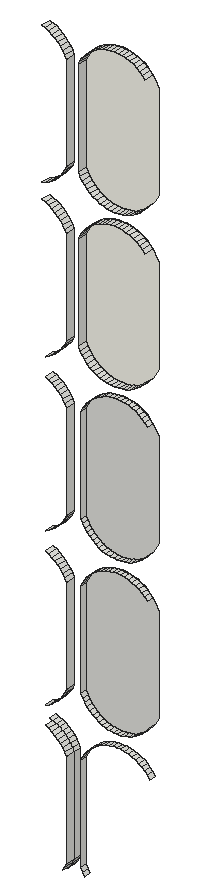
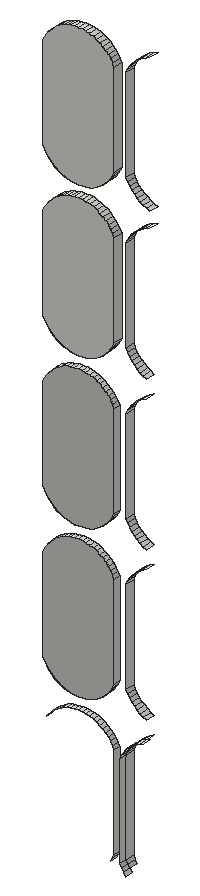
# SketchUp Ruby script. Lengths in inches.
U = 1.inch
M = Sketchup.active_model
def pt(a) = Geom::Point3d.new(a.map { |v| v * U })
def face(e, loops, mat)
  f = e.add_face(loops[0].map { |a| pt(a) })
  loops[1..].each { |l| e.add_face(l.map { |a| pt(a) }).erase! }
  f.material = f.back_material = mat if mat
  f
end
# faces: each face lists its corners as indices into pts; further lists are holes
def faces(e, pts, list, mat = nil) = list.each { |f| face(e, (f[0].is_a?(Array) ? f : [f]).map { |l| l.map { |i| pts[i] } }, mat) }
# xy, xz, yz: faces in a plane at the given z, y or x. An outline is a flat list of corners, or four numbers for a rectangle; further outlines are holes
def ring(l) = l.size == 4 ? [[l[0], l[1]], [l[2], l[1]], [l[2], l[3]], [l[0], l[3]]] : l.each_slice(2).to_a
def flat(e, list, mat, &to3) = list.each { |f| face(e, (f[0].is_a?(Array) ? f : [f]).map { |l| ring(l).map { |u, v| to3.(u, v) } }, mat) }
def xy(e, z, list, mat = nil) = flat(e, list, mat) { |x, y| [x, y, z] }
def xz(e, y, list, mat = nil) = flat(e, list, mat) { |x, z| [x, y, z] }
def yz(e, x, list, mat = nil) = flat(e, list, mat) { |y, z| [x, y, z] }
def lines(e, pts, list) = list.each { |a, b| e.add_line(pt(pts[a]), pt(pts[b])) }
# prism: a flat outline (further loops are holes) pulled along v
def prism(e, loops, v, mat = nil)
  f = face(e, loops, mat); d = Geom::Vector3d.new(v.map { |x| x * U })
  f.pushpull(f.normal.samedirection?(d) ? d.length : -d.length)
end
def box(e, o, s, mat = nil) = prism(e, [[o, [o[0] + s[0], o[1], o[2]], [o[0] + s[0], o[1] + s[1], o[2]], [o[0], o[1] + s[1], o[2]]]], [0, 0, s[2]], mat)
def at(x, y, z, deg = 0) = Geom::Transformation.translation(pt([x, y, z])) * Geom::Transformation.rotation(ORIGIN, Z_AXIS, deg.degrees)
def axes(o, x, y, z) = Geom::Transformation.new([*x, 0, *y, 0, *z, 0, *pt(o).to_a, 1])
def part(name) = M.definitions.add(name)
# library, detail: a bought-in or finely detailed component or shape, given as its bounding box
def library(name, o, s) = part(name).tap { |d| box(d.entities, o, s) }
def detail(e, o, s) = box(e.add_group.entities, o, s)
def put(e, d, t, mat = nil) = e.add_instance(d, t).tap { |i| i.material = mat if mat }
def group(e, t, mat = nil) = e.add_group.tap { |g| g.transformation = t; g.material = mat if mat }.entities
root = M.entities
M.materials.add("Tafisa-Gardenia-or-Gardenia-PM775-4K").color = [246, 245, 235]
xz(root,138.79,[[89.53,63,89.85,63.02,90.17,63.0625,90.48,63.14,90.78,63.25,91.07,63.38,91.35,63.55,91.61,63.73,91.84,63.95,92.0625,64.18,92.25,64.4375,92.42,64.71,92.5625,65,92.5625,73,92.42,73.29,92.25,73.5625,92.0625,73.82,91.84,74.05,91.61,74.27,91.35,74.45,91.07,74.62,90.78,74.75,90.48,74.86,90.17,74.9375,89.85,74.98,89.53,75,89.21,74.98,88.89,74.9375,88.58,74.86,88.28,74.75,87.99,74.62,87.72,74.45,87.46,74.27,87.22,74.05,87,73.82,86.81,73.5625,86.64,73.29,86.5,73,86.5,65,86.64,64.71,86.81,64.4375,87,64.18,87.22,63.95,87.46,63.73,87.72,63.55,87.99,63.38,88.28,63.25,88.58,63.14,88.89,63.0625,89.21,63.02],[89.53,76,89.85,76.02,90.17,76.0625,90.48,76.14,90.78,76.25,91.07,76.38,91.35,76.55,91.61,76.73,91.84,76.95,92.0625,77.18,92.25,77.4375,92.42,77.71,92.5625,78,92.5625,86,92.42,86.29,92.25,86.5625,92.0625,86.82,91.84,87.05,91.61,87.27,91.35,87.45,91.07,87.62,90.78,87.75,90.48,87.86,90.17,87.9375,89.85,87.98,89.53,88,89.21,87.98,88.89,87.9375,88.58,87.86,88.28,87.75,87.99,87.62,87.72,87.45,87.46,87.27,87.22,87.05,87,86.82,86.81,86.5625,86.64,86.29,86.5,86,86.5,78,86.64,77.71,86.81,77.4375,87,77.18,87.22,76.95,87.46,76.73,87.72,76.55,87.99,76.38,88.28,76.25,88.58,76.14,88.89,76.0625,89.21,76.02]])
xz(root,138.79,[[89.53,89,89.85,89.02,90.17,89.0625,90.48,89.14,90.78,89.25,91.07,89.38,91.35,89.55,91.61,89.73,91.84,89.95,92.0625,90.18,92.25,90.4375,92.42,90.71,92.5625,91,92.5625,99,92.42,99.29,92.25,99.5625,92.0625,99.82,91.84,100.05,91.61,100.27,91.35,100.45,91.07,100.62,90.78,100.75,90.48,100.86,90.17,100.9375,89.85,100.98,89.53,101,89.21,100.98,88.89,100.9375,88.58,100.86,88.28,100.75,87.99,100.62,87.72,100.45,87.46,100.27,87.22,100.05,87,99.82,86.81,99.5625,86.64,99.29,86.5,99,86.5,91,86.64,90.71,86.81,90.4375,87,90.18,87.22,89.95,87.46,89.73,87.72,89.55,87.99,89.38,88.28,89.25,88.58,89.14,88.89,89.0625,89.21,89.02],[89.53,102,89.85,102.02,90.17,102.0625,90.48,102.14,90.78,102.25,91.07,102.38,91.35,102.55,91.61,102.73,91.84,102.95,92.0625,103.18,92.25,103.4375,92.42,103.71,92.5625,104,92.5625,112,92.42,112.29,92.25,112.5625,92.0625,112.82,91.84,113.05,91.61,113.27,91.35,113.45,91.07,113.62,90.78,113.75,90.48,113.86,90.17,113.9375,89.85,113.98,89.53,114,89.21,113.98,88.89,113.9375,88.58,113.86,88.28,113.75,87.99,113.62,87.72,113.45,87.46,113.27,87.22,113.05,87,112.82,86.81,112.5625,86.64,112.29,86.5,112,86.5,104,86.64,103.71,86.81,103.4375,87,103.18,87.22,102.95,87.46,102.73,87.72,102.55,87.99,102.38,88.28,102.25,88.58,102.14,88.89,102.0625,89.21,102.02]],"Tafisa-Gardenia-or-Gardenia-PM775-4K")
yz(root,85.5,[[138,52,138.79,60],[138.79,52,139.4375,60],[138,65,138.79,73],[138,78,138.79,86],[138,91,138.79,99],
  [138,104,138.79,112]])
yz(root,86.5,[[138.25,52,138.79,60],[138.25,65,138.79,73],[138.25,78,138.79,86],[138,91,138.79,99],[138,104,138.79,112]])
p = [[85.01,139.4375,51.18],[85.01,138.79,51.18],[85.2,138.79,51.44],[85.2,139.4375,51.44],[85.36,138.79,51.71],[85.2,138,51.44],
  [85.36,138,51.71],[86.81,138.79,51.4375],[86.64,138.79,51.71],[86.64,138.25,51.71],[86.81,138.25,51.4375],[85.36,139.4375,51.71],
  [85.5,138.79,52],[85.5,138,52],[86.5,138.79,52],[86.5,138.25,52],[85.5,139.4375,52],[85.36,138.79,60.29],
  [85.5,138.79,60],[85.5,138,60],[85.36,138,60.29],[86.5,138.79,60],[86.64,138.79,60.29],[86.64,138.25,60.29],
  [86.5,138.25,60],[85.5,139.4375,60],[85.36,139.4375,60.29],[85.2,138.79,60.56],[85.2,138,60.56],[86.81,138.79,60.5625],
  [86.81,138.25,60.5625],[85.2,139.4375,60.56],[85.01,138.79,60.82],[85.01,138,60.82],[87,138.79,60.82],[87,138.25,60.82],
  [92.0625,138.79,60.82],[92.25,138.79,60.5625],[92.25,138.25,60.5625],[92.0625,138.25,60.82],[85.01,139.4375,60.82],[84.79,138.79,61.05],
  [84.79,138,61.05],[87.22,138.79,61.05],[87.22,138.25,61.05],[91.84,138.79,61.05],[91.84,138.25,61.05],[84.79,139.4375,61.05],
  [84.56,138.79,61.26],[84.56,138,61.26],[87.46,138.79,61.27],[87.46,138.25,61.27],[91.61,138.79,61.27],[91.61,138.25,61.27],
  [84.56,139.4375,61.26],[84.3,138.79,61.45],[84.3,138,61.45],[87.72,138.79,61.45],[87.72,138.25,61.45],[91.35,138.79,61.45],
  [91.35,138.25,61.45],[84.3,139.4375,61.45],[84.03,138.79,61.62],[84.03,138,61.62],[87.99,138.79,61.62],[87.99,138.25,61.62],
  [91.07,138.79,61.62],[91.07,138.25,61.62],[84.03,139.4375,61.62],[83.74,138.79,61.75],[83.74,138,61.75],[88.28,138.79,61.75],
  [88.28,138.25,61.75],[90.78,138.79,61.75],[90.78,138.25,61.75],[83.74,139.4375,61.75],[88.58,138.79,61.86],[88.58,138.25,61.86],
  [90.48,138.79,61.86],[90.48,138.25,61.86],[83.44,138.79,61.86],[83.44,139.4375,61.86],[88.89,138.79,61.9375],[88.89,138.25,61.9375],
  [89.21,138.79,61.98],[89.21,138.25,61.98],[89.02,138.25,61.96],[89.85,138.79,61.98],[90.17,138.79,61.9375],[90.17,138.25,61.9375],
  [89.85,138.25,61.98],[89.53,138.79,62],[89.53,138.25,62],[89.21,138.79,63.02],[88.89,138.79,63.0625],[88.89,138.25,63.0625],
  [89.02,138.25,63.04],[89.21,138.25,63.02],[89.53,138.79,63],[89.53,138.25,63],[89.85,138.79,63.02],[89.85,138.25,63.02],
  [90.17,138.79,63.0625],[90.17,138.25,63.0625],[88.58,138.79,63.14],[88.28,138.79,63.25],[88.28,138.25,63.25],[88.58,138.25,63.14],
  [88.78,138.25,63.09],[90.48,138.79,63.14],[90.48,138.25,63.14],[90.78,138.79,63.25],[90.78,138.25,63.25],[84.03,138.79,63.38],
  [83.74,138.79,63.25],[83.74,138,63.25],[84.03,138,63.38],[87.99,138.79,63.38],[87.99,138.25,63.38],[91.07,138.79,63.38],
  [91.07,138.25,63.38],[84.3,138.79,63.55],[84.3,138,63.55],[87.72,138.79,63.55],[87.72,138.25,63.55],[91.35,138.79,63.55],
  [91.35,138.25,63.55],[84.56,138.79,63.74],[84.56,138,63.74],[87.46,138.79,63.73],[87.46,138.25,63.73],[91.61,138.79,63.73],
  [91.61,138.25,63.73],[84.79,138.79,63.95],[84.79,138,63.95],[87.22,138.79,63.95],[87.22,138.25,63.95],[91.84,138.79,63.95],
  [91.84,138.25,63.95],[85.01,138.79,64.18],[85.01,138,64.18],[87,138.79,64.18],[87,138.25,64.18],[92.0625,138.79,64.18],
  [92.0625,138.25,64.18],[85.2,138.79,64.44],[85.2,138,64.44],[86.81,138.79,64.4375],[86.81,138.25,64.4375],[92.25,138.79,64.4375],
  [92.25,138.25,64.4375],[85.36,138.79,64.71],[85.36,138,64.71],[86.64,138.79,64.71],[86.64,138.25,64.71],[85.5,138.79,65],
  [85.5,138,65],[86.5,138.79,65],[86.5,138.25,65],[85.36,138.79,73.29],[85.5,138.79,73],[85.5,138,73],
  [85.36,138,73.29],[86.5,138.79,73],[86.64,138.79,73.29],[86.64,138.25,73.29],[86.5,138.25,73],[85.2,138.79,73.56],
  [85.2,138,73.56],[86.81,138.79,73.5625],[86.81,138.25,73.5625],[85.01,138.79,73.82],[85.01,138,73.82],[87,138.79,73.82],
  [87,138.25,73.82],[84.79,138.79,74.05],[84.79,138,74.05],[87.22,138.79,74.05],[87.22,138.25,74.05],[91.84,138.79,74.05],
  [92.0625,138.79,73.82],[92.0625,138.25,73.82],[91.84,138.25,74.05],[84.56,138.79,74.26],[84.56,138,74.26],[87.46,138.79,74.27],
  [87.46,138.25,74.27],[91.61,138.79,74.27],[91.61,138.25,74.27],[84.3,138.79,74.45],[84.3,138,74.45],[87.72,138.79,74.45],
  [87.72,138.25,74.45],[91.35,138.79,74.45],[91.35,138.25,74.45],[84.03,138.79,74.62],[84.03,138,74.62],[87.99,138.79,74.62],
  [87.99,138.25,74.62],[91.07,138.79,74.62],[91.07,138.25,74.62],[83.74,138.79,74.75],[83.74,138,74.75],[88.28,138.79,74.75],
  [88.28,138.25,74.75],[90.78,138.79,74.75],[90.78,138.25,74.75],[88.58,138.79,74.86],[88.58,138.25,74.86],[90.48,138.79,74.86],
  [90.48,138.25,74.86],[88.89,138.79,74.9375],[88.89,138.25,74.9375],[89.21,138.79,74.98],[89.21,138.25,74.98],[89.02,138.25,74.96],
  [89.85,138.79,74.98],[90.17,138.79,74.9375],[90.17,138.25,74.9375],[89.85,138.25,74.98],[89.53,138.79,75],[89.53,138.25,75],
  [89.21,138.79,76.02],[88.89,138.79,76.0625],[88.89,138.25,76.0625],[89.02,138.25,76.04],[89.21,138.25,76.02],[89.53,138.79,76],
  [89.53,138.25,76],[89.85,138.79,76.02],[89.85,138.25,76.02],[90.17,138.79,76.0625],[90.17,138.25,76.0625],[88.58,138.79,76.14],
  [88.28,138.79,76.25],[88.28,138.25,76.25],[88.58,138.25,76.14],[90.48,138.79,76.14],[90.48,138.25,76.14],[90.78,138.79,76.25],
  [90.78,138.25,76.25],[84.03,138.79,76.38],[83.74,138.79,76.25],[83.74,138,76.25],[84.03,138,76.38],[87.99,138.79,76.38],
  [87.99,138.25,76.38],[91.07,138.79,76.38],[91.07,138.25,76.38],[84.3,138.79,76.55],[84.3,138,76.55],[87.72,138.79,76.55],
  [87.72,138.25,76.55],[91.35,138.79,76.55],[91.35,138.25,76.55],[84.56,138.79,76.74],[84.56,138,76.74],[87.46,138.79,76.73],
  [87.46,138.25,76.73],[91.61,138.79,76.73],[91.61,138.25,76.73],[84.79,138.79,76.95],[84.79,138,76.95],[87.22,138.79,76.95],
  [87.22,138.25,76.95],[91.84,138.79,76.95],[91.84,138.25,76.95],[85.01,138.79,77.18],[85.01,138,77.18],[87,138.79,77.18],
  [87,138.25,77.18],[92.0625,138.79,77.18],[92.0625,138.25,77.18],[85.2,138.79,77.44],[85.2,138,77.44],[86.81,138.79,77.4375],
  [86.81,138.25,77.4375],[85.36,138.79,77.71],[85.36,138,77.71],[86.64,138.79,77.71],[86.64,138.25,77.71],[85.5,138.79,78],
  [85.5,138,78],[86.5,138.79,78],[86.5,138.25,78],[85.36,138.79,86.29],[85.5,138.79,86],[85.5,138,86],
  [85.36,138,86.29],[86.5,138.79,86],[86.64,138.79,86.29],[86.64,138.25,86.29],[86.5,138.25,86],[85.2,138.79,86.56],
  [85.2,138,86.56],[86.81,138.79,86.5625],[86.81,138.25,86.5625],[85.01,138.79,86.82],[85.01,138,86.82],[87,138.79,86.82],
  [87,138.25,86.82],[84.79,138.79,87.05],[84.79,138,87.05],[87.22,138.79,87.05],[87.22,138.25,87.05],[91.84,138.79,87.05],
  [92.0625,138.79,86.82],[92.0625,138.25,86.82],[91.84,138.25,87.05],[84.56,138.79,87.26],[84.56,138,87.26],[87.46,138.79,87.27],
  [87.46,138.25,87.27],[91.61,138.79,87.27],[91.61,138.25,87.27],[84.3,138.79,87.45],[84.3,138,87.45],[87.72,138.79,87.45],
  [87.72,138.25,87.45],[91.35,138.79,87.45],[91.35,138.25,87.45],[84.03,138.79,87.62],[84.03,138,87.62],[87.99,138.79,87.62],
  [87.99,138.25,87.62],[91.07,138.79,87.62],[91.07,138.25,87.62],[83.74,138.79,87.75],[83.74,138,87.75],[88.28,138.79,87.75],
  [88.28,138.25,87.75],[90.78,138.79,87.75],[90.78,138.25,87.75],[88.58,138.79,87.86],[88.58,138.25,87.86],[90.48,138.79,87.86],
  [90.48,138.25,87.86],[88.89,138.79,87.9375],[88.89,138.25,87.9375],[89.21,138.79,87.98],[89.21,138.25,87.98],[89.85,138.79,87.98],
  [90.17,138.79,87.9375],[90.17,138.25,87.9375],[89.85,138.25,87.98],[89.53,138.79,88],[89.53,138.25,88],[89.21,138.79,89.02],
  [88.89,138.79,89.0625],[88.89,138,89.0625],[89.21,138,89.02],[89.53,138.79,89],[89.53,138,89],[89.85,138.79,89.02],
  [89.85,138,89.02],[90.17,138.79,89.0625],[90.17,138,89.0625],[88.58,138.79,89.14],[88.28,138.79,89.25],[88.28,138,89.25],
  [88.58,138,89.14],[90.48,138.79,89.14],[90.48,138,89.14],[90.78,138.79,89.25],[90.78,138,89.25],[84.03,138.79,89.38],
  [83.74,138.79,89.25],[83.74,138,89.25],[84.03,138,89.38],[87.99,138.79,89.38],[87.99,138,89.38],[91.07,138.79,89.38],
  [91.07,138,89.38],[84.3,138.79,89.55],[84.3,138,89.55],[87.72,138.79,89.55],[87.72,138,89.55],[91.35,138.79,89.55],
  [91.35,138,89.55],[84.56,138.79,89.74],[84.56,138,89.74],[87.46,138.79,89.73],[87.46,138,89.73],[91.61,138.79,89.73],
  [91.61,138,89.73],[84.79,138.79,89.95],[84.79,138,89.95],[87.22,138.79,89.95],[87.22,138,89.95],[91.84,138.79,89.95],
  [91.84,138,89.95],[85.01,138.79,90.18],[85.01,138,90.18],[87,138.79,90.18],[87,138,90.18],[92.0625,138.79,90.18],
  [92.0625,138,90.18],[85.2,138.79,90.44],[85.2,138,90.44],[86.81,138.79,90.4375],[86.81,138,90.4375],[85.36,138.79,90.71],
  [85.36,138,90.71],[86.64,138.79,90.71],[86.64,138,90.71],[85.5,138.79,91],[85.5,138,91],[86.5,138.79,91],
  [86.5,138,91],[85.36,138.79,99.29],[85.5,138.79,99],[85.5,138,99],[85.36,138,99.29],[86.5,138.79,99],
  [86.64,138.79,99.29],[86.64,138,99.29],[86.5,138,99],[85.2,138.79,99.56],[85.2,138,99.56],[86.81,138.79,99.5625],
  [86.81,138,99.5625],[85.01,138.79,99.82],[85.01,138,99.82],[87,138.79,99.82],[87,138,99.82],[84.79,138.79,100.05],
  [84.79,138,100.05],[87.22,138.79,100.05],[87.22,138,100.05],[91.84,138.79,100.05],[92.0625,138.79,99.82],[92.0625,138,99.82],
  [91.84,138,100.05],[84.56,138.79,100.26],[84.56,138,100.26],[87.46,138.79,100.27],[87.46,138,100.27],[91.61,138.79,100.27],
  [91.61,138,100.27],[84.3,138.79,100.45],[84.3,138,100.45],[87.72,138.79,100.45],[87.72,138,100.45],[91.35,138.79,100.45],
  [91.35,138,100.45],[84.03,138.79,100.62],[84.03,138,100.62],[87.99,138.79,100.62],[87.99,138,100.62],[91.07,138.79,100.62],
  [91.07,138,100.62],[83.74,138.79,100.75],[83.74,138,100.75],[88.28,138.79,100.75],[88.28,138,100.75],[90.78,138.79,100.75],
  [90.78,138,100.75],[83.44,138.79,100.86],[83.44,138,100.86],[88.58,138.79,100.86],[88.58,138,100.86],[90.48,138.79,100.86],
  [90.48,138,100.86],[88.89,138.79,100.9375],[88.89,138,100.9375],[89.21,138.79,100.98],[89.21,138,100.98],[89.85,138.79,100.98],
  [90.17,138.79,100.9375],[90.17,138,100.9375],[89.85,138,100.98],[89.53,138.79,101],[89.53,138,101],[89.21,138.79,102.02],
  [88.89,138.79,102.0625],[88.89,138,102.0625],[89.21,138,102.02],[89.53,138.79,102],[89.53,138,102],[89.85,138.79,102.02],
  [89.85,138,102.02],[90.17,138.79,102.0625],[90.17,138,102.0625],[83.74,138.79,102.25],[83.44,138.79,102.14],[83.44,138,102.14],
  [83.74,138,102.25],[88.58,138.79,102.14],[88.28,138.79,102.25],[88.28,138,102.25],[88.58,138,102.14],[90.48,138.79,102.14],
  [90.48,138,102.14],[90.78,138.79,102.25],[90.78,138,102.25],[84.03,138.79,102.38],[84.03,138,102.38],[87.99,138.79,102.38],
  [87.99,138,102.38],[91.07,138.79,102.38],[91.07,138,102.38],[84.3,138.79,102.55],[84.3,138,102.55],[87.72,138.79,102.55],
  [87.72,138,102.55],[91.35,138.79,102.55],[91.35,138,102.55],[84.56,138.79,102.74],[84.56,138,102.74],[87.46,138.79,102.73],
  [87.46,138,102.73],[91.61,138.79,102.73],[91.61,138,102.73],[84.79,138.79,102.95],[84.79,138,102.95],[87.22,138.79,102.95],
  [87.22,138,102.95],[91.84,138.79,102.95],[91.84,138,102.95],[85.01,138.79,103.18],[85.01,138,103.18],[87,138.79,103.18],
  [87,138,103.18],[92.0625,138.79,103.18],[92.0625,138,103.18],[85.2,138.79,103.44],[85.2,138,103.44],[86.81,138.79,103.4375],
  [86.81,138,103.4375],[85.36,138.79,103.71],[85.36,138,103.71],[86.64,138.79,103.71],[86.64,138,103.71],[85.5,138.79,104],
  [85.5,138,104],[86.5,138.79,104],[86.5,138,104],[85.36,138.79,112.29],[85.5,138.79,112],[85.5,138,112],
  [85.36,138,112.29],[86.5,138.79,112],[86.64,138.79,112.29],[86.64,138,112.29],[86.5,138,112],[85.2,138.79,112.56],
  [85.2,138,112.56],[86.81,138.79,112.5625],[86.81,138,112.5625],[85.01,138.79,112.82],[85.01,138,112.82],[87,138.79,112.82],
  [87,138,112.82],[84.79,138.79,113.05],[84.79,138,113.05],[87.22,138.79,113.05],[87.22,138,113.05],[91.84,138.79,113.05],
  [92.0625,138.79,112.82],[92.0625,138,112.82],[91.84,138,113.05],[84.56,138.79,113.26],[84.56,138,113.26],[87.46,138.79,113.27],
  [87.46,138,113.27],[91.61,138.79,113.27],[91.61,138,113.27],[84.3,138.79,113.45],[84.3,138,113.45],[87.72,138.79,113.45],
  [87.72,138,113.45],[91.35,138.79,113.45],[91.35,138,113.45],[84.03,138.79,113.62],[84.03,138,113.62],[87.99,138.79,113.62],
  [87.99,138,113.62],[91.07,138.79,113.62],[91.07,138,113.62],[83.74,138.79,113.75],[83.74,138,113.75],[88.28,138.79,113.75],
  [88.28,138,113.75],[90.78,138.79,113.75],[90.78,138,113.75],[83.44,138.79,113.86],[83.44,138,113.86],[88.58,138.79,113.86],
  [88.58,138,113.86],[90.48,138.79,113.86],[90.48,138,113.86],[88.89,138.79,113.9375],[88.89,138,113.9375],[89.21,138.79,113.98],
  [89.21,138,113.98],[89.85,138.79,113.98],[90.17,138.79,113.9375],[90.17,138,113.9375],[89.85,138,113.98],[89.53,138.79,114],
  [89.53,138,114]]
faces(root,p,[[0,1,2,3],[4,2,5,6],[7,8,9,10],[3,2,4,11],[12,4,6,13],[8,14,15,9],[11,4,12,16],[17,18,19,20],
  [21,22,23,24],[25,18,17,26],[27,17,20,28],[22,29,30,23],[26,17,27,31],[32,27,28,33],[29,34,35,30],[36,37,38,39],
  [31,27,32,40],[41,32,33,42],[34,43,44,35],[45,36,39,46],[40,32,41,47],[48,41,42,49],[43,50,51,44],[52,45,46,53],
  [47,41,48,54],[55,48,49,56],[50,57,58,51],[59,52,53,60],[54,48,55,61],[62,55,56,63],[57,64,65,58],[66,59,60,67],
  [61,55,62,68],[69,62,63,70],[64,71,72,65],[73,66,67,74],[68,62,69,75],[71,76,77,72],[78,73,74,79],[75,69,80,81],
  [76,82,83,77],[82,84,85,86,83],[87,88,89,90],[88,78,79,89],[84,91,92,85],[91,87,90,92],[93,94,95,96,97],[98,93,97,99],
  [100,98,99,101],[102,100,101,103],[104,105,106,107],[94,104,107,108,95],[109,102,103,110],[111,109,110,112],[113,114,115,116],[105,117,118,106],
  [119,111,112,120],[121,113,116,122],[117,123,124,118],[125,119,120,126],[127,121,122,128],[123,129,130,124],[131,125,126,132],[133,127,128,134],
  [129,135,136,130],[137,131,132,138],[139,133,134,140],[135,141,142,136],[143,137,138,144],[145,139,140,146],[141,147,148,142],[149,143,144,150],
  [151,145,146,152],[147,153,154,148],[155,151,152,156],[153,157,158,154],[159,160,161,162],[163,164,165,166],[167,159,162,168],[164,169,170,165],
  [171,167,168,172],[169,173,174,170],[175,171,172,176],[173,177,178,174],[179,180,181,182],[183,175,176,184],[177,185,186,178],[187,179,182,188],
  [189,183,184,190],[185,191,192,186],[193,187,188,194],[195,189,190,196],[191,197,198,192],[199,193,194,200],[201,195,196,202],[197,203,204,198],
  [205,199,200,206],[203,207,208,204],[209,205,206,210],[207,211,212,208],[211,213,214,215,212],[216,217,218,219],[217,209,210,218],[213,220,221,214],
  [220,216,219,221],[222,223,224,225,226],[227,222,226,228],[229,227,228,230],[231,229,230,232],[233,234,235,236],[223,233,236,224],[237,231,232,238],
  [239,237,238,240],[241,242,243,244],[234,245,246,235],[247,239,240,248],[249,241,244,250],[245,251,252,246],[253,247,248,254],[255,249,250,256],
  [251,257,258,252],[259,253,254,260],[261,255,256,262],[257,263,264,258],[265,259,260,266],[267,261,262,268],[263,269,270,264],[271,265,266,272],
  [273,267,268,274],[269,275,276,270],[277,273,274,278],[275,279,280,276],[281,277,278,282],[279,283,284,280],[285,286,287,288],[289,290,291,292],
  [293,285,288,294],[290,295,296,291],[297,293,294,298],[295,299,300,296],[301,297,298,302],[299,303,304,300],[305,306,307,308],[309,301,302,310],
  [303,311,312,304],[313,305,308,314],[315,309,310,316],[311,317,318,312],[319,313,314,320],[321,315,316,322],[317,323,324,318],[325,319,320,326],
  [327,321,322,328],[323,329,330,324],[331,325,326,332],[329,333,334,330],[335,331,332,336],[333,337,338,334],[337,339,340,338],[341,342,343,344],
  [342,335,336,343],[339,345,346,340],[345,341,344,346],[347,348,349,350],[351,347,350,352],[353,351,352,354],[355,353,354,356],[357,358,359,360],
  [348,357,360,349],[361,355,356,362],[363,361,362,364],[365,366,367,368],[358,369,370,359],[371,363,364,372],[373,365,368,374],[369,375,376,370],
  [377,371,372,378],[379,373,374,380],[375,381,382,376],[383,377,378,384],[385,379,380,386],[381,387,388,382],[389,383,384,390],[391,385,386,392],
  [387,393,394,388],[395,389,390,396],[397,391,392,398],[393,399,400,394],[401,397,398,402],[399,403,404,400],[405,401,402,406],[403,407,408,404],
  [409,410,411,412],[413,414,415,416],[417,409,412,418],[414,419,420,415],[421,417,418,422],[419,423,424,420],[425,421,422,426],[423,427,428,424],
  [429,430,431,432],[433,425,426,434],[427,435,436,428],[437,429,432,438],[439,433,434,440],[435,441,442,436],[443,437,438,444],[445,439,440,446],
  [441,447,448,442],[449,443,444,450],[451,445,446,452],[447,453,454,448],[455,449,450,456],[457,451,452,458],[453,459,460,454],[461,455,456,462],
  [459,463,464,460],[463,465,466,464],[467,468,469,470],[468,461,462,469],[465,471,472,466],[471,467,470,472],[473,474,475,476],[477,473,476,478],
  [479,477,478,480],[481,479,480,482],[483,484,485,486],[487,488,489,490],[474,487,490,475],[491,481,482,492],[493,491,492,494],[495,483,486,496],
  [488,497,498,489],[499,493,494,500],[501,495,496,502],[497,503,504,498],[505,499,500,506],[507,501,502,508],[503,509,510,504],[511,505,506,512],
  [513,507,508,514],[509,515,516,510],[517,511,512,518],[519,513,514,520],[515,521,522,516],[523,517,518,524],[525,519,520,526],[521,527,528,522],
  [529,525,526,530],[527,531,532,528],[533,529,530,534],[531,535,536,532],[537,538,539,540],[541,542,543,544],[545,537,540,546],[542,547,548,543],
  [549,545,546,550],[547,551,552,548],[553,549,550,554],[551,555,556,552],[557,558,559,560],[561,553,554,562],[555,563,564,556],[565,557,560,566],
  [567,561,562,568],[563,569,570,564],[571,565,566,572],[573,567,568,574],[569,575,576,570],[577,571,572,578],[579,573,574,580],[575,581,582,576],
  [583,577,578,584],[585,579,580,586],[581,587,588,582],[589,583,584,590],[587,591,592,588],[591,593,594,592],[595,596,597,598],[596,589,590,597],
  [593,599,600,594],[599,595,598,600]])
